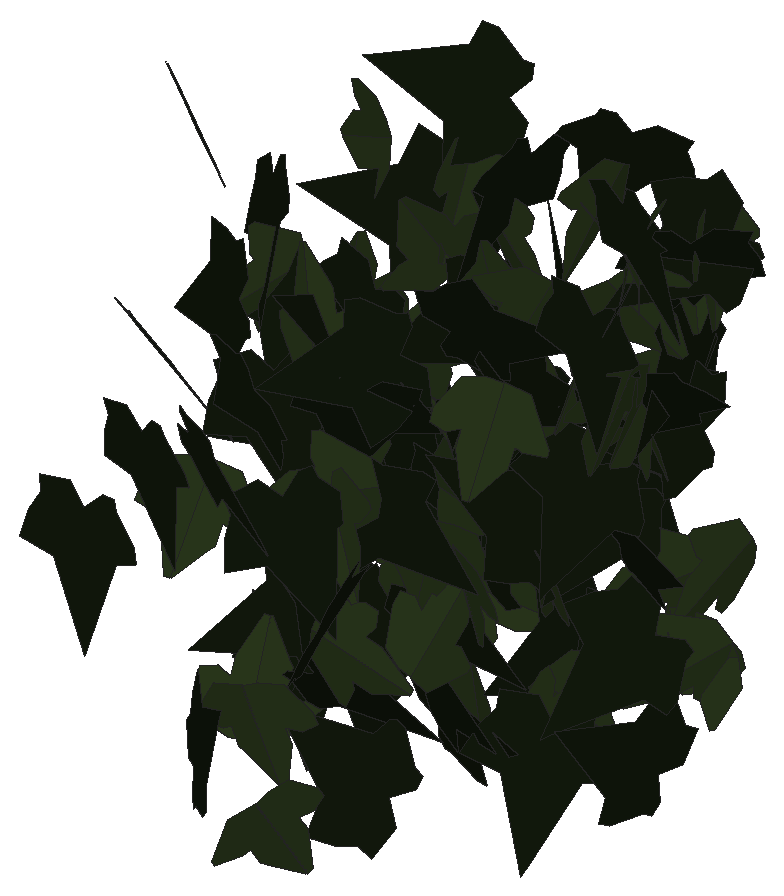
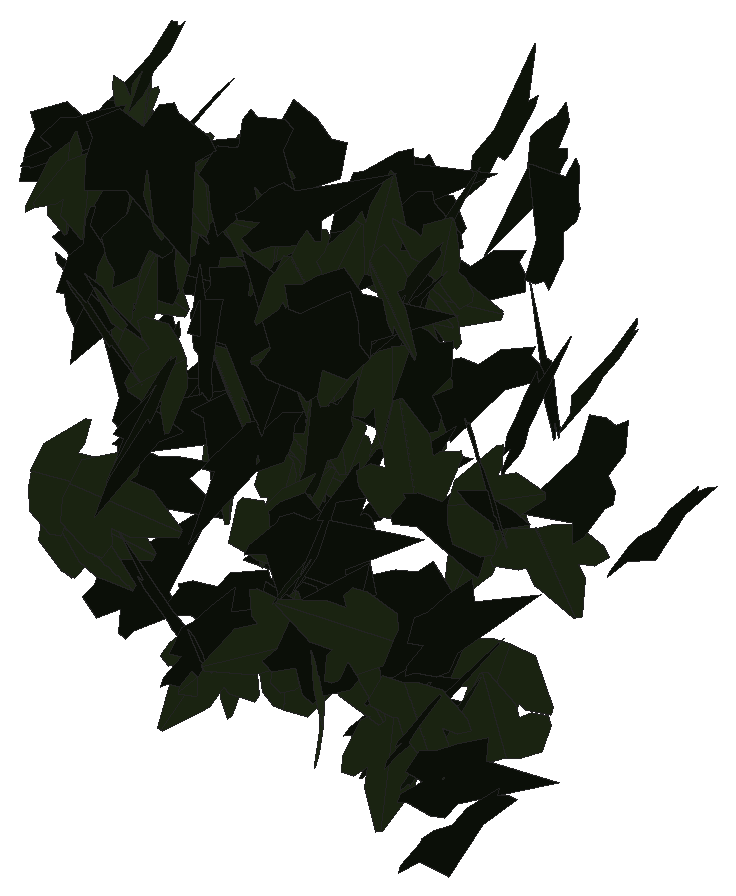
# SketchUp Ruby script. Lengths in inches.
U = 1.inch
M = Sketchup.active_model
def pt(a) = Geom::Point3d.new(a.map { |v| v * U })
def face(e, loops, mat)
  f = e.add_face(loops[0].map { |a| pt(a) })
  loops[1..].each { |l| e.add_face(l.map { |a| pt(a) }).erase! }
  f.material = f.back_material = mat if mat
  f
end
# faces: each face lists its corners as indices into pts; further lists are holes
def faces(e, pts, list, mat = nil) = list.each { |f| face(e, (f[0].is_a?(Array) ? f : [f]).map { |l| l.map { |i| pts[i] } }, mat) }
# xy, xz, yz: faces in a plane at the given z, y or x. An outline is a flat list of corners, or four numbers for a rectangle; further outlines are holes
def ring(l) = l.size == 4 ? [[l[0], l[1]], [l[2], l[1]], [l[2], l[3]], [l[0], l[3]]] : l.each_slice(2).to_a
def flat(e, list, mat, &to3) = list.each { |f| face(e, (f[0].is_a?(Array) ? f : [f]).map { |l| ring(l).map { |u, v| to3.(u, v) } }, mat) }
def xy(e, z, list, mat = nil) = flat(e, list, mat) { |x, y| [x, y, z] }
def xz(e, y, list, mat = nil) = flat(e, list, mat) { |x, z| [x, y, z] }
def yz(e, x, list, mat = nil) = flat(e, list, mat) { |y, z| [x, y, z] }
def lines(e, pts, list) = list.each { |a, b| e.add_line(pt(pts[a]), pt(pts[b])) }
# prism: a flat outline (further loops are holes) pulled along v
def prism(e, loops, v, mat = nil)
  f = face(e, loops, mat); d = Geom::Vector3d.new(v.map { |x| x * U })
  f.pushpull(f.normal.samedirection?(d) ? d.length : -d.length)
end
def box(e, o, s, mat = nil) = prism(e, [[o, [o[0] + s[0], o[1], o[2]], [o[0] + s[0], o[1] + s[1], o[2]], [o[0], o[1] + s[1], o[2]]]], [0, 0, s[2]], mat)
def at(x, y, z, deg = 0) = Geom::Transformation.translation(pt([x, y, z])) * Geom::Transformation.rotation(ORIGIN, Z_AXIS, deg.degrees)
def axes(o, x, y, z) = Geom::Transformation.new([*x, 0, *y, 0, *z, 0, *pt(o).to_a, 1])
def part(name) = M.definitions.add(name)
# library, detail: a bought-in or finely detailed component or shape, given as its bounding box
def library(name, o, s) = part(name).tap { |d| box(d.entities, o, s) }
def detail(e, o, s) = box(e.add_group.entities, o, s)
def put(e, d, t, mat = nil) = e.add_instance(d, t).tap { |i| i.material = mat if mat }
def group(e, t, mat = nil) = e.add_group.tap { |g| g.transformation = t; g.material = mat if mat }.entities
root = M.entities
M.materials.add("efeu1").color = [18, 25, 13]
M.materials.add("efeu2").color = [43, 57, 29]
c1 = part("ivyleaf_9")
p = [[1.54,2.16,1.25],[1.36,2.04,1.19],[-0.21,0.99,0.68],[-0.71,1.11,0.82],[-0.85,0.86,0.67],[-0.8,0.17,0.21],
  [-0.9,-0.01,0.1],[-0.67,-0.16,-0.02],[-0.08,-0.08,-0.05],[-0.03,-0.6,-0.4],[0.65,-0.88,-0.66],[0.83,-0.6,-0.49],
  [1.29,-0.42,-0.43],[1.8125,-0.07,-0.26],[1.21,0.44,0.15]]
faces(c1.entities,p,[[0,1,2,3,4,5,6,7,8,9,10,11,12,13,14]],"efeu1")
c2 = part("ivyleaf_10")
p = [[0,0.5,-0.03],[-0.0625,2.02,-0.43],[-0.19,2.01,-0.46],[-0.54,1.05,-0.29],[-0.52,0.625,-0.18],[-0.83,0.76,-0.28],
  [-1.16,0.64,-0.33],[-1.15,0.33,-0.24],[-0.77,-0.39,0.02],[-0.3,-0.51,0.16],[0.04,-0.48,0.23],[-0.02,2.01,-0.4375],
  [-0.06,2.01,-0.43],[0.04,-0.49,0.23],[0.67,-0.49,0.14],[1.38,0.36,-0.2],[1.375,0.51,-0.24],[0.81,0.65,-0.19],
  [0.62,0.59,-0.15],[0.6,1.09,-0.28],[0.5,1.23,-0.31]]
faces(c2.entities,p,[[0,1,2,3,4,5,6,7,8,9,10],[11,12,0,13,14,15,16,17,18,19,20]],"efeu2")
put(root,c1,axes([40.88,221.85,211.85],[-0.24399,0.00193,-0.43642],[0.43108,-0.07701,-0.24134],[-0.06815,-0.49403,0.03592]))
put(root,c1,axes([40.7,220.01,210.96],[0.40696,-0.26515,0.11867],[0.10044,-0.06323,-0.48571],[0.27257,0.41917,0.0018]))
put(root,c2,axes([41.25,221.57,211.09],[-0.01857,-0.0853,0.49232],[0.00173,-0.49267,-0.08529],[0.49965,-0.00146,0.0186]))
put(root,c1,axes([41.09,218.63,209.6],[0.02948,-0.49677,0.04851],[0.00663,-0.0482,-0.49763],[0.49909,0.02998,0.00374]))
put(root,c1,axes([41.48,221.98,209.54],[-0.1597,-0.20183,0.42867],[-0.28136,-0.32358,-0.25717],[0.38123,-0.32336,-0.01022]))
put(root,c1,axes([41.49,220.53,211.33],[-0.06203,-0.08947,0.488],[-0.10525,-0.47824,-0.10105],[0.48484,-0.11526,0.04049]))
put(root,c1,axes([41.52,221.65,211.05],[-0.33285,-0.34297,-0.1469],[0.10194,0.10577,-0.47793],[0.35891,-0.34811,-0.00048]))
put(root,c1,axes([41.82,221.55,207.57],[-0.31226,-0.19395,0.33894],[-0.29092,-0.17397,-0.36756],[0.26051,-0.42675,-0.0042]))
put(root,c1,axes([41.45,221.61,207.18],[-0.00618,-0.49886,-0.0332],[0.00271,0.03316,-0.49889],[0.49995,-0.00635,0.0023]))
put(root,c1,axes([41.29,219.98,213.7],[0.27522,-0.07541,-0.41057],[0.40279,-0.08114,0.28492],[-0.1096,-0.48758,0.01608]))
put(root,c2,axes([41.71,219.72,209.67],[0.44304,0.19804,-0.12039],[-0.11119,-0.04625,-0.48528],[-0.20334,0.45677,0.00306]))
put(root,c1,axes([41.91,221.78,208.18],[0.1307,-0.44571,-0.18509],[0.05493,-0.17677,0.46447],[-0.47948,-0.14174,0.00276]))
put(root,c2,axes([41.91,221.68,208.58],[0.49551,0.02677,-0.06125],[-0.0613,-0.00074,-0.49623],[-0.02666,0.49928,0.00255]))
put(root,c2,axes([42.09,221.52,210.95],[-0.16533,-0.47156,-0.01729],[-0.00575,-0.0163,0.4997],[-0.47184,0.16543,-0.00003]))
put(root,c1,axes([41.96,221.31,207.79],[0.01729,-0.37814,0.32666],[0.06087,-0.32283,-0.37693],[0.49598,0.0528,0.03487]))
put(root,c2,axes([42.17,219.88,207.17],[0.39262,0.28672,-0.11678],[0.08733,0.07836,0.48604],[0.29702,-0.40205,0.01145]))
put(root,c1,axes([42.07,218.33,210.94],[0.18376,-0.45004,0.11705],[0.04445,-0.10828,-0.48611],[0.46288,0.18906,0.00022]))
put(root,c2,axes([42.63,221.3,213.22],[0.18112,-0.16453,-0.43603],[-0.31212,0.30457,-0.24457],[0.34609,0.36078,0.00763]))
put(root,c2,axes([42.64,221.14,207.64],[-0.25517,-0.42104,-0.08724],[0.05057,0.07135,-0.49229],[0.427,-0.26006,0.00617]))
put(root,c2,axes([42.63,219.35,207.7],[-0.47041,-0.13826,-0.09799],[0.09721,0.01667,-0.49018],[0.13881,-0.48022,0.01119]))
put(root,c1,axes([42.86,220.86,210.46],[-0.16217,-0.34901,0.31921],[-0.12074,-0.29572,-0.38467],[0.4573,-0.20184,0.01163]))
put(root,c1,axes([42.9,221.09,207.87],[-0.19328,-0.31581,0.33602],[-0.1542,-0.2991,-0.36981],[0.43459,-0.24658,0.01823]))
put(root,c1,axes([42.53,220.69,211.59],[0.38956,-0.20756,0.23486],[0.20534,-0.11404,-0.44139],[0.2368,0.44035,-0.00361]))
put(root,c1,axes([42.77,219.53,211.33],[-0.07818,-0.44044,-0.22339],[0.07056,0.21389,-0.4464],[0.48878,-0.10132,0.02872]))
put(root,c2,axes([43.02,220.64,211.67],[-0.15011,-0.47358,-0.05645],[0.01881,0.05326,-0.4968],[0.47656,-0.15127,0.00183]))
put(root,c1,axes([43.36,221.43,212.55],[-0.23662,-0.00217,0.44046],[-0.43964,-0.02941,-0.23633],[0.02694,-0.49913,0.01201]))
put(root,c2,axes([43.34,221.31,208.64],[-0.34332,-0.13046,0.33928],[-0.31817,-0.11785,-0.36726],[0.1758,-0.46807,-0.0021]))
put(root,c2,axes([42.8,221.33,208.89],[0.15014,0.04445,-0.47485],[0.44433,0.16783,0.15621],[0.17328,-0.46889,0.0109]))
put(root,c1,axes([42.9,220.71,207.48],[0.15188,-0.42191,0.22118],[0.07314,-0.20874,-0.44841],[0.47073,0.16857,-0.00169]))
put(root,c2,axes([43.05,221.87,208.08],[-0.03615,0.04016,-0.49707],[0.19118,-0.45918,-0.051],[-0.46059,-0.19375,0.01784]))
put(root,c1,axes([43.16,221.08,210.55],[0.23746,-0.27921,-0.34008],[-0.20118,0.27479,-0.36608],[0.39133,0.3107,0.01815]))
put(root,c1,axes([43.7,221.49,209.71],[-0.19611,0.03493,0.45861],[-0.45927,0.01205,-0.1973],[-0.02484,-0.49863,0.02736]))
put(root,c1,axes([43.24,220.49,212.01],[-0.03642,-0.43708,0.24008],[0.00229,-0.24086,-0.43816],[0.49867,-0.03082,0.01955]))
put(root,c1,axes([43.6,221.52,208.36],[0.26168,-0.14043,0.40225],[-0.35675,0.18585,0.29697],[-0.23292,-0.44243,-0.00293]))
put(root,c2,axes([43.53,219.24,212.08],[0.46099,-0.03673,0.1901],[-0.18817,0.03062,0.46223],[-0.0456,-0.49771,0.01441]))
put(root,c1,axes([43.74,221.9,213.79],[-0.15211,-0.39774,-0.26204],[-0.08907,-0.24647,0.42581],[-0.4679,0.17622,0.00413]))
put(root,c1,axes([43.37,221.6,210.16],[-0.05557,-0.44086,-0.22925],[0.03192,0.22704,-0.44434],[0.49588,-0.06402,0.00291]))
put(root,c1,axes([43.22,221.64,212.14],[-0.07817,-0.06603,0.48942],[0.43411,-0.24543,0.03622],[0.23545,0.43059,0.0957]))
put(root,c1,axes([43.93,219.79,206.92],[-0.38607,-0.18495,-0.25835],[-0.22665,-0.12461,0.4279],[-0.22267,0.44751,0.01238]))
put(root,c1,axes([43.29,219.6,208.12],[0.46736,0.11259,0.13747],[0.13348,0.0329,-0.48073],[-0.11729,0.48605,0.0007]))
put(root,c2,axes([43.68,219.43,210.51],[-0.00515,-0.00463,0.49995],[-0.19821,0.45903,0.00221],[-0.45901,-0.19817,-0.00657]))
put(root,c2,axes([43.75,221.05,212.35],[-0.27061,-0.31287,-0.28086],[-0.17376,-0.22093,0.41352],[-0.38285,0.32141,0.01085]))
put(root,c2,axes([43.625,221.56,213.15],[0.05273,0.42147,-0.26378],[-0.06038,-0.25787,-0.42409],[-0.49353,0.07658,0.0237]))
put(root,c1,axes([43.39,221.3125,210.81],[0.09079,-0.30093,0.38885],[0.13758,-0.36408,-0.31388],[0.47205,0.16399,0.01669]))
put(root,c1,axes([43.67,219.5625,212],[0.23958,-0.43408,-0.06466],[0.04512,-0.04892,0.49555],[-0.43654,-0.24328,0.01573]))
put(root,c2,axes([43.86,221.75,209.875],[0.12317,0.35604,0.32873],[-0.10234,-0.31242,0.37672],[0.47366,-0.16009,-0.00409]))
put(root,c1,axes([43.5,221.35,209.7],[0.18523,-0.44503,0.13279],[0.05162,-0.12235,-0.48204],[0.46155,0.19229,0.00062]))
put(root,c2,axes([43.76,221.39,208.48],[0.13331,0.07925,0.47534],[0.34279,0.33105,-0.15134],[-0.33871,0.36623,0.03393]))
put(root,c2,axes([43.89,220.47,211.67],[-0.01325,-0.00856,-0.49975],[0.3011,0.3989,-0.01482],[0.39896,-0.30134,-0.00542]))
put(root,c1,axes([43.98,216.74,212.27],[0.42007,-0.21008,-0.17148],[-0.14943,0.08453,-0.4696],[0.2263,0.44578,0.00824]))
put(root,c2,axes([44.55,218.52,211.14],[-0.05372,-0.07417,0.49154],[-0.31995,-0.37323,-0.09128],[0.38045,-0.32435,-0.00736]))
put(root,c2,axes([44.28,220.94,210.05],[-0.39243,0.30965,0.01075],[-0.00895,0.00601,-0.49988],[-0.3097,-0.39253,0.00083]))
put(root,c1,axes([44.13,217.48,212.55],[0.33622,-0.28315,-0.23828],[0.183,-0.15261,0.43957],[-0.32166,-0.3828,0.00101]))
put(root,c1,axes([44.22,221.42,210.82],[0.14807,-0.31401,-0.35982],[-0.12113,0.3397,-0.34631],[0.46195,0.18973,0.02453]))
put(root,c2,axes([44.48,219.16,211.84],[-0.48883,0.09666,-0.04125],[-0.04246,-0.00214,0.49819],[0.09613,0.49056,0.0103]))
put(root,c1,axes([44.49,221.0625,212.26],[0.31373,0.25132,-0.29734],[-0.22962,-0.18893,-0.40197],[-0.3144,0.38877,-0.00312]))
put(root,c1,axes([44.04,220.2,209.04],[0.05688,0.03832,-0.49527],[0.43311,0.2403,0.06834],[0.24326,-0.43679,-0.00586]))
put(root,c2,axes([44.46,220.61,207.39],[-0.49644,0.04692,0.03668],[0.03636,-0.00516,0.49865],[0.04717,0.49777,0.00171]))
put(root,c1,axes([44.28,217.8,211.21],[-0.01892,-0.3973,-0.30298],[0.02384,0.30213,-0.39768],[0.49907,-0.0295,0.00751]))
put(root,c1,axes([44.56,220.85,212.19],[0.01351,-0.20801,-0.45448],[0.03262,-0.45331,0.20844],[-0.49875,-0.03528,0.00132]))
put(root,c1,axes([44.57,218.65,212.14],[0.2341,0.3417,-0.28008],[-0.17556,-0.21892,-0.41383],[-0.40544,0.29209,0.01748]))
put(root,c2,axes([44.4375,217.3,207.97],[-0.23624,-0.36887,-0.24108],[0.12907,0.20362,-0.43804],[0.42134,-0.2692,-0.00099]))
put(root,c1,axes([44.28,216.4,208.89],[-0.04925,0.17067,0.46738],[0.10985,-0.45435,0.17749],[0.48529,0.12017,0.00726]))
put(root,c2,axes([44.57,220.82,212.07],[-0.36017,-0.32643,-0.11715],[-0.08571,-0.07987,0.48608],[-0.33606,0.37022,0.00158]))
put(root,c1,axes([44.13,220.16,208.22],[0.20948,-0.00427,-0.45398],[0.45261,0.04106,0.20846],[0.0355,-0.49829,0.02107]))
put(root,c2,axes([44.2,220.45,210.08],[-0.09539,0.03262,0.48973],[0.48333,-0.08058,0.09951],[0.08542,0.49238,-0.01616]))
put(root,c1,axes([44.72,218.97,212.49],[-0.02225,-0.27156,-0.41924],[-0.03494,-0.41778,0.27247],[-0.49828,0.04142,-0.00038]))
put(root,c1,axes([44.23,220.34,207.62],[0.13167,-0.13293,0.46367],[0.32086,-0.33473,-0.18708],[0.36015,0.34682,-0.00284]))
put(root,c2,axes([44.4375,218.28,211.06],[0.38769,-0.03037,0.31428],[0.31291,-0.02952,-0.38886],[0.04217,0.4982,-0.00388]))
put(root,c1,axes([44.8,220.98,213.85],[-0.12946,0.25624,-0.40937],[0.1796,-0.36788,-0.28707],[-0.44831,-0.22137,0.00321]))
put(root,c1,axes([44.45,218.84,210.86],[-0.01103,-0.09643,-0.49049],[0.2601,0.41786,-0.088],[0.42688,-0.25709,0.04094]))
put(root,c2,axes([44.91,219.375,210.36],[-0.43792,-0.20024,0.13466],[-0.12108,-0.05901,-0.48151],[0.20873,-0.45434,0.00319]))
put(root,c2,axes([44.93,221.08,211.22],[0.30714,-0.27371,-0.28416],[-0.21817,0.18222,-0.41134],[0.32873,0.37667,-0.0075]))
put(root,c1,axes([44.96,221.47,211.6],[0.06672,-0.16978,0.46554],[-0.11312,0.45212,0.18109],[-0.48245,-0.12949,0.02192]))
put(root,c1,axes([44.9,221.78,208.12],[-0.14444,-0.25266,0.40657],[-0.20959,-0.34843,-0.29098],[0.43036,-0.25448,-0.00525]))
put(root,c2,axes([44.55,220.97,212.98],[-0.14078,0.13495,-0.4604],[0.35424,-0.29435,-0.1946],[-0.32357,-0.38098,-0.01274]))
put(root,c2,axes([44.55,218.26,209.55],[-0.12508,0.00358,-0.48409],[0.46453,-0.13986,-0.12106],[-0.13627,-0.48003,0.03167]))
put(root,c2,axes([44.85,219.22,209.09],[0.13212,0.28734,-0.38727],[0.13546,0.36326,0.31574],[0.46281,-0.18835,0.01814]))
put(root,c1,axes([45.06,220.45,210.77],[0.33443,0.35034,-0.12417],[-0.09472,-0.08118,-0.48419],[-0.35942,0.34737,0.01207]))
put(root,c2,axes([44.97,221.17,207.89],[-0.22569,-0.31874,-0.31219],[0.19751,0.24234,-0.39021],[0.40007,-0.29945,0.01652]))
put(root,c2,axes([45.12,219.55,210.04],[-0.42882,0.24511,0.07766],[-0.06649,0.04016,-0.49393],[-0.24837,-0.43394,-0.00185]))
put(root,c2,axes([45.1,220.7,207.625],[-0.00037,-0.031,-0.49904],[0.07639,0.49318,-0.03069],[0.49413,-0.07626,0.00437]))
put(root,c1,axes([45.22,221.5,208.17],[-0.28757,0.33936,0.22834],[0.15084,-0.17146,0.4448],[0.3802,0.32471,-0.00377]))
put(root,c1,axes([45.52,220.2,210.3],[-0.03776,-0.49405,-0.06701],[-0.00508,-0.06682,0.49549],[-0.49855,0.0381,0.00003]))
put(root,c2,axes([45.6,220.23,212.93],[-0.35849,-0.26566,0.22563],[-0.18621,-0.12764,-0.44613],[0.29464,-0.4039,-0.00742]))
put(root,c1,axes([45.57,221.63,214.1],[0.18494,0.27659,-0.37322],[-0.22408,-0.29877,-0.33245],[-0.40692,0.29023,0.01344]))
put(root,c2,axes([45.42,221.46,213.57],[0.03458,-0.41971,0.26954],[0.0433,-0.26664,-0.42075],[0.49692,0.05244,0.01791]))
put(root,c2,axes([45.59,220.2,209.94],[-0.36577,0.20664,0.27113],[-0.23662,0.13237,-0.4201],[-0.2454,-0.43564,0.00096]))
put(root,c1,axes([45.35,221.55,211.33],[0.36868,-0.21674,-0.25904],[-0.22158,0.13423,-0.42765],[0.25492,0.43013,0.00292]))
put(root,c1,axes([45.1,219.48,212.6875],[0.23104,-0.05162,0.4404],[0.43206,-0.08548,-0.23668],[0.09973,0.48993,0.00511]))
put(root,c2,axes([45.32,221.53,211.36],[-0.27865,0.20258,-0.36237],[0.30419,-0.19737,-0.34425],[-0.28253,-0.41231,-0.01325]))
put(root,c1,axes([45.61,220.32,208.01],[-0.2771,-0.3982,-0.12104],[0.06648,0.1012,-0.48512],[0.41085,-0.28495,-0.00314]))
put(root,c1,axes([45.32,219.78,212.04],[0.09125,0.1427,-0.47043],[0.26818,0.38655,0.16928],[0.41201,-0.28322,-0.00599]))
put(root,c1,axes([45.84,216.4,210.9375],[-0.19509,0.19302,-0.41795],[-0.29091,0.30012,0.2744],[0.3568,0.35024,-0.0048]))
put(root,c1,axes([45.57,221.31,210.71],[0.16234,-0.27463,-0.385],[-0.16959,0.34617,-0.31844],[0.44146,0.23397,0.01925]))
put(root,c1,axes([45.77,221.27,210.33],[-0.23815,-0.40353,0.17451],[-0.08092,-0.15485,-0.46848],[0.43213,-0.25138,0.00845]))
put(root,c1,axes([45.54,221.6,212.74],[0.43476,-0.20024,-0.14454],[0.13065,-0.06185,0.47865],[-0.20957,-0.45396,-0.00146]))
put(root,c2,axes([46.3,221.61,209.46],[-0.12054,-0.16015,0.45806],[-0.28128,-0.36154,-0.20042],[0.39541,-0.30601,-0.00293]))
put(root,c2,axes([45.97,220.49,212.29],[-0.09594,0.18179,-0.45579],[0.03556,-0.46063,-0.1912],[-0.48942,-0.0691,0.07546]))
put(root,c2,axes([46.06,218.86,212.44],[0.48307,0.10703,-0.07205],[-0.07024,-0.01606,-0.49478],[-0.10822,0.48815,-0.00048]))
put(root,c2,axes([46.37,220.92,211.12],[-0.42614,0.22553,-0.13246],[-0.11703,0.06205,0.48214],[0.23391,0.44191,-0.0001]))
put(root,c2,axes([46.46,220.55,213.36],[0.01625,0.08787,-0.49195],[-0.20345,0.45074,0.07378],[0.45645,0.19778,0.0504]))
put(root,c2,axes([46.38,220.98,211.92],[-0.05327,-0.34133,0.36146],[-0.05862,-0.35668,-0.34546],[0.49369,-0.07918,-0.00202]))
put(root,c1,axes([46.5,221.58,211.8],[-0.45367,0.1831,-0.10324],[0.09578,-0.03852,-0.48923],[-0.18711,-0.46367,-0.00012]))
put(root,c1,axes([46.46,220.4375,213.18],[-0.32989,0.28307,-0.24707],[0.17907,-0.1706,-0.43454],[-0.33032,-0.37519,0.01118]))
put(root,c1,axes([46.55,220.7,209.21],[-0.39587,-0.27402,0.13489],[-0.11107,-0.07655,-0.48146],[0.28451,-0.41116,-0.00027]))
put(root,c2,axes([46.33,220.55,213.08],[-0.35938,-0.22262,-0.26699],[0.2205,0.15088,-0.42263],[0.26874,-0.42151,-0.01027]))
put(root,c2,axes([46.28,220.89,213.48],[-0.08841,-0.16745,-0.46276],[0.14499,-0.45816,0.13809],[-0.47028,-0.10977,0.12957]))
put(root,c1,axes([46.57,220.74,207.68],[0.01934,0.028,0.49884],[-0.36364,-0.34156,0.03327],[0.34263,-0.36408,0.00715]))
put(root,c2,axes([46.41,221.53,213.36],[0.08714,0.49104,-0.03591],[-0.00584,-0.03544,-0.49871],[-0.49231,0.08733,-0.00044]))
put(root,c1,axes([46.5,219.9375,211.42],[-0.20991,-0.44495,0.08917],[-0.02863,-0.08507,-0.49188],[0.4529,-0.21161,0.01024]))
put(root,c1,axes([46.9,221.04,211.52],[-0.39887,0.20306,0.22287],[-0.20021,0.09796,-0.44757],[-0.22543,-0.44628,0.00316]))
put(root,c2,axes([46.86,221.34,208.8],[0.2186,-0.07018,-0.44417],[-0.42577,0.12661,-0.22955],[0.14469,0.47859,-0.00441]))
put(root,c1,axes([46.49,220.61,212.02],[0.41467,0.27353,-0.05684],[-0.05004,-0.02737,-0.49674],[-0.27486,0.41765,0.00467]))
put(root,c1,axes([46.5,221.46,212.34],[-0.03073,0.03634,-0.49773],[0.32951,-0.37304,-0.04758],[-0.3748,-0.33094,-0.00102]))
put(root,c1,axes([46.75,221.09,213.51],[0.14795,0.38532,-0.28221],[-0.09712,-0.26499,-0.41273],[-0.46763,0.17695,-0.00357]))
put(root,c1,axes([46.42,219.96,213.06],[0.06913,-0.47698,0.13306],[0.03411,-0.12945,-0.48175],[0.49402,0.07569,0.01464]))
put(root,c2,axes([46.51,220.65,211.81],[-0.00598,0.0765,-0.49408],[0.06857,-0.48932,-0.0766],[-0.49524,-0.06868,-0.00464]))
put(root,c2,axes([46.85,221.27,208.89],[-0.13311,-0.2158,0.43094],[-0.22565,-0.36714,-0.25355],[0.42587,-0.26199,0.00035]))
put(root,c2,axes([46.7,220.05,212.35],[-0.00935,-0.4878,0.10939],[-0.00566,-0.1093,-0.48787],[0.49988,-0.01036,-0.00348]))
put(root,c2,axes([46.63,221.65,213.42],[-0.05814,0.4916,-0.07033],[-0.04983,-0.07623,-0.49164],[-0.4941,-0.05016,0.05786]))
put(root,c1,axes([46.38,220.52,214.05],[0.27198,-0.41571,0.05665],[0.03103,-0.04739,-0.49678],[0.41841,0.27374,0.00002]))
put(root,c1,axes([46.82,221.56,213.47],[-0.30331,-0.27594,0.28611],[-0.1976,-0.2076,-0.4097],[0.3449,-0.3616,0.01689]))
put(root,c2,axes([46.67,221.85,209.66],[0.00053,-0.24398,0.43643],[0.06094,-0.43315,-0.24222],[0.49627,0.05345,0.02928]))
put(root,c1,axes([46.31,220.5625,210.24],[0.1162,-0.1813,0.45125],[0.28822,-0.34802,-0.21404],[0.3917,0.30986,0.02363]))
